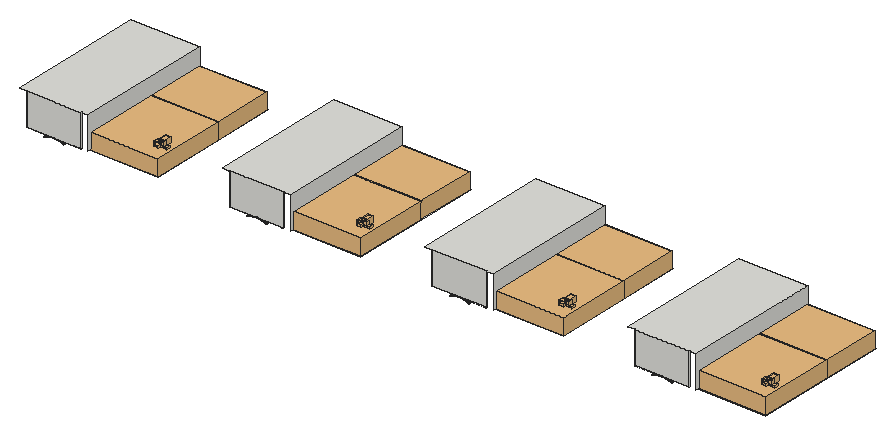
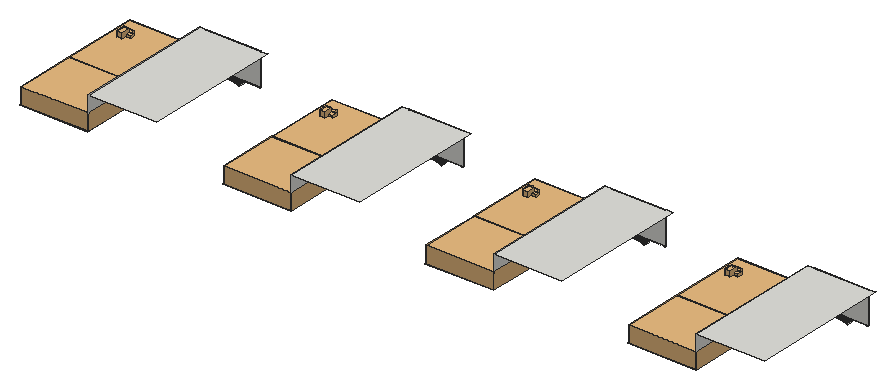
# SketchUp Ruby script. Lengths in inches.
U = 1.inch
M = Sketchup.active_model
def pt(a) = Geom::Point3d.new(a.map { |v| v * U })
def face(e, loops, mat)
  f = e.add_face(loops[0].map { |a| pt(a) })
  loops[1..].each { |l| e.add_face(l.map { |a| pt(a) }).erase! }
  f.material = f.back_material = mat if mat
  f
end
# faces: each face lists its corners as indices into pts; further lists are holes
def faces(e, pts, list, mat = nil) = list.each { |f| face(e, (f[0].is_a?(Array) ? f : [f]).map { |l| l.map { |i| pts[i] } }, mat) }
# xy, xz, yz: faces in a plane at the given z, y or x. An outline is a flat list of corners, or four numbers for a rectangle; further outlines are holes
def ring(l) = l.size == 4 ? [[l[0], l[1]], [l[2], l[1]], [l[2], l[3]], [l[0], l[3]]] : l.each_slice(2).to_a
def flat(e, list, mat, &to3) = list.each { |f| face(e, (f[0].is_a?(Array) ? f : [f]).map { |l| ring(l).map { |u, v| to3.(u, v) } }, mat) }
def xy(e, z, list, mat = nil) = flat(e, list, mat) { |x, y| [x, y, z] }
def xz(e, y, list, mat = nil) = flat(e, list, mat) { |x, z| [x, y, z] }
def yz(e, x, list, mat = nil) = flat(e, list, mat) { |y, z| [x, y, z] }
def lines(e, pts, list) = list.each { |a, b| e.add_line(pt(pts[a]), pt(pts[b])) }
# prism: a flat outline (further loops are holes) pulled along v
def prism(e, loops, v, mat = nil)
  f = face(e, loops, mat); d = Geom::Vector3d.new(v.map { |x| x * U })
  f.pushpull(f.normal.samedirection?(d) ? d.length : -d.length)
end
def box(e, o, s, mat = nil) = prism(e, [[o, [o[0] + s[0], o[1], o[2]], [o[0] + s[0], o[1] + s[1], o[2]], [o[0], o[1] + s[1], o[2]]]], [0, 0, s[2]], mat)
def at(x, y, z, deg = 0) = Geom::Transformation.translation(pt([x, y, z])) * Geom::Transformation.rotation(ORIGIN, Z_AXIS, deg.degrees)
def axes(o, x, y, z) = Geom::Transformation.new([*x, 0, *y, 0, *z, 0, *pt(o).to_a, 1])
def part(name) = M.definitions.add(name)
# library, detail: a bought-in or finely detailed component or shape, given as its bounding box
def library(name, o, s) = part(name).tap { |d| box(d.entities, o, s) }
def detail(e, o, s) = box(e.add_group.entities, o, s)
def put(e, d, t, mat = nil) = e.add_instance(d, t).tap { |i| i.material = mat if mat }
def group(e, t, mat = nil) = e.add_group.tap { |g| g.transformation = t; g.material = mat if mat }.entities
root = M.entities
M.materials.add("POT_TEXTURE_1").color = [172, 172, 172]
M.materials.add("soil1").color = [68, 55, 47]
c1 = library("Group\#96",[-662.41,217.3,320.04],[397.32,658.3,1732.06])
c2 = library("Group\#98",[-299.2,181.55,262.58],[360.65,735.71,1258.34])
c3 = library("Group\#93",[-1038.76,656.55,345.34],[733.18,460.51,2065.7])
c4 = library("Group\#91",[-445.29,890.31,329.28],[284.3,304.08,2023.29])
c5 = library("Group\#94",[-733.48,439.625,202.64],[456.28,533.12,1536.78])
c6 = library("Group\#97",[-455.56,899.32,410.78],[341.21,610.33,1581.5])
c7 = library("Group\#90",[-516.34,626.77,-4.5625],[517.73,515.95,418.98])
c8 = library("Group\#95",[-249.24,914.85,310.18],[345.55,647.95,1307.93])
c9 = library("Group\#92",[-277.97,488.68,287.26],[362.84,405.94,1768.54])
c10 = library("Group\#89",[-468.76,669.89,380.1875],[424.36,427.47,41.99])
c11 = part("Potted broadleaf plant")
put(c11.entities,c1,at(1038.76,-181.55,4.5625))
put(c11.entities,c2,at(1038.76,-181.55,4.5625))
put(c11.entities,c3,at(1038.76,-181.55,4.5625))
put(c11.entities,c4,at(1038.76,-181.55,4.5625))
put(c11.entities,c5,at(1038.76,-181.55,4.5625))
put(c11.entities,c6,at(1038.76,-181.55,4.5625))
put(c11.entities,c7,at(1038.76,-181.55,4.5625),"POT_TEXTURE_1")
put(c11.entities,c8,at(1038.76,-181.55,4.5625))
put(c11.entities,c9,at(1038.76,-181.55,4.5625))
put(c11.entities,c10,at(1038.76,-181.55,4.5625),"soil1")
c12 = library("Glass Railing\#2",[-0.5,-0.75,0],[149.1875,165.51,35.5])
c13 = library("Glass Railing\#3",[-148.4375,-0.5,0],[149.1875,132.1875,35.5])
xy(root,270.89,[[159.1,224.6875,215.92,225.16],[222.08,224.6875,278.75,225.16],[603.1,224.6875,659.92,225.16],[666.08,224.6875,722.75,225.16],[1047.1,224.6875,1103.92,225.16],
  [1110.08,224.6875,1166.75,225.16],[1491.1,224.6875,1547.92,225.16],[1554.08,224.6875,1610.75,225.16]])
xy(root,271,[[218.38,224.6875,219,225.16],[219,224.6875,219.61,225.16],[662.38,224.6875,663,225.16],[663,224.6875,663.61,225.16],[1106.38,224.6875,1107,225.16],
  [1107,224.6875,1107.61,225.16],[1550.38,224.6875,1551,225.16],[1551,224.6875,1551.61,225.16],[218.38,225.16,219,236.25],[219,225.16,219.61,236.25],
  [662.38,225.16,663,236.25],[663,225.16,663.61,236.25],[1106.38,225.16,1107,236.25],[1107,225.16,1107.61,236.25],[1550.38,225.16,1551,236.25],
  [1551,225.16,1551.61,236.25],[294,229.25,444,529.25],[738,229.25,888,529.25],[1182,229.25,1332,529.25],[1626,229.25,1776,529.25]])
xy(root,271.37,[[159.1,224.6875,215.92,225.16],[215.92,224.6875,222.08,225.16],[222.08,224.6875,278.75,225.16],[603.1,224.6875,659.92,225.16],[659.92,224.6875,666.08,225.16],
  [666.08,224.6875,722.75,225.16],[1047.1,224.6875,1103.92,225.16],[1103.92,224.6875,1110.08,225.16],[1110.08,224.6875,1166.75,225.16],[1491.1,224.6875,1547.92,225.16],
  [1547.92,224.6875,1554.08,225.16],[1554.08,224.6875,1610.75,225.16]])
xy(root,342,[[144,224.6875,158.625,224.6875,158.625,225.16,159.1,225.16,159.1,224.6875,278.75,224.6875,278.75,225.16,279.22,225.16,279.22,224.6875,294,224.6875,294,529.25,144,529.25],[588,224.6875,602.625,224.6875,602.625,225.16,603.1,225.16,603.1,224.6875,722.75,224.6875,722.75,225.16,723.22,225.16,723.22,224.6875,738,224.6875,738,529.25,588,529.25],[1032,224.6875,1046.625,224.6875,1046.625,225.16,1047.1,225.16,1047.1,224.6875,1166.75,224.6875,1166.75,225.16,1167.22,225.16,1167.22,224.6875,1182,224.6875,1182,529.25,1032,529.25],[1476,224.6875,1490.625,224.6875,1490.625,225.16,1491.1,225.16,1491.1,224.6875,1610.75,224.6875,1610.75,225.16,1611.22,225.16,1611.22,224.6875,1626,224.6875,1626,529.25,1476,529.25]])
xz(root,224.6875,[[215.92,270.89,222.08,270.89,222.05,270.9,220.83,270.96,219.61,271,218.38,271,217.77,270.98,217.15,270.96,216.53,270.93],[659.92,270.89,666.08,270.89,666.05,270.9,664.83,270.96,663.61,271,662.38,271,661.77,270.98,661.15,270.96,660.53,270.93],[1103.92,270.89,1110.08,270.89,1110.05,270.9,1108.83,270.96,1107.61,271,1106.38,271,1105.77,270.98,1105.15,270.96,1104.53,270.93],[1547.92,270.89,1554.08,270.89,1554.05,270.9,1552.83,270.96,1551.61,271,1550.38,271,1549.77,270.98,1549.15,270.96,1548.53,270.93],[159.1,271.37,278.75,342],
  [603.1,271.37,722.75,342],[1047.1,271.37,1166.75,342],[1491.1,271.37,1610.75,342]])
yz(root,159.1,[[224.6875,271.37,225.16,342]])
yz(root,278.75,[[224.6875,271.37,225.16,342]])
yz(root,294,[[224.6875,271,529.25,342]])
yz(root,603.1,[[224.6875,271.37,225.16,342]])
yz(root,722.75,[[224.6875,271.37,225.16,342]])
yz(root,738,[[224.6875,271,529.25,342]])
yz(root,1047.1,[[224.6875,271.37,225.16,342]])
yz(root,1166.75,[[224.6875,271.37,225.16,342]])
yz(root,1182,[[224.6875,271,529.25,342]])
yz(root,1491.1,[[224.6875,271.37,225.16,342]])
yz(root,1610.75,[[224.6875,271.37,225.16,342]])
yz(root,1626,[[224.6875,271,529.25,342]])
p = [[241.22,236.25,265.14],[241.22,224.6875,265.14],[240.68,224.6875,265.43],[240.68,236.25,265.43],[685.22,236.25,265.14],[685.22,224.6875,265.14],
  [684.68,224.6875,265.43],[684.68,236.25,265.43],[1129.22,236.25,265.14],[1129.22,224.6875,265.14],[1128.68,224.6875,265.43],[1128.68,236.25,265.43],
  [1573.22,236.25,265.14],[1573.22,224.6875,265.14],[1572.68,224.6875,265.43],[1572.68,236.25,265.43],[197.69,236.25,265.62],[197.69,224.6875,265.62],
  [197.15,224.6875,265.32],[197.15,236.25,265.32],[641.69,236.25,265.62],[641.69,224.6875,265.62],[641.15,224.6875,265.32],[641.15,236.25,265.32],
  [1085.69,236.25,265.62],[1085.69,224.6875,265.62],[1085.15,224.6875,265.32],[1085.15,236.25,265.32],[1529.69,236.25,265.62],[1529.69,224.6875,265.62],
  [1529.15,224.6875,265.32],[1529.15,236.25,265.32],[240.15,224.6875,265.72],[240.15,236.25,265.72],[684.15,224.6875,265.72],[684.15,236.25,265.72],
  [1128.15,224.6875,265.72],[1128.15,236.25,265.72],[1572.15,224.6875,265.72],[1572.15,236.25,265.72],[198.24,236.25,265.91],[198.24,224.6875,265.91],
  [642.24,236.25,265.91],[642.24,224.6875,265.91],[1086.24,236.25,265.91],[1086.24,224.6875,265.91],[1530.24,236.25,265.91],[1530.24,224.6875,265.91],
  [239.6,224.6875,266.01],[239.6,236.25,266.01],[683.6,224.6875,266.01],[683.6,236.25,266.01],[1127.6,224.6875,266.01],[1127.6,236.25,266.01],
  [1571.6,224.6875,266.01],[1571.6,236.25,266.01],[198.79,236.25,266.1875],[198.79,224.6875,266.1875],[642.79,236.25,266.1875],[642.79,224.6875,266.1875],
  [1086.79,236.25,266.1875],[1086.79,224.6875,266.1875],[1530.79,236.25,266.1875],[1530.79,224.6875,266.1875],[239.06,224.6875,266.28],[239.06,236.25,266.28],
  [683.06,224.6875,266.28],[683.06,236.25,266.28],[1127.06,224.6875,266.28],[1127.06,236.25,266.28],[1571.06,224.6875,266.28],[1571.06,236.25,266.28],
  [199.34,236.25,266.46],[199.34,224.6875,266.46],[643.34,236.25,266.46],[643.34,224.6875,266.46],[1087.34,236.25,266.46],[1087.34,224.6875,266.46],
  [1531.34,236.25,266.46],[1531.34,224.6875,266.46],[238.51,224.6875,266.55],[238.51,236.25,266.55],[682.51,224.6875,266.55],[682.51,236.25,266.55],
  [1126.51,224.6875,266.55],[1126.51,236.25,266.55],[1570.51,224.6875,266.55],[1570.51,236.25,266.55],[199.89,236.25,266.73],[199.89,224.6875,266.73],
  [643.89,236.25,266.73],[643.89,224.6875,266.73],[1087.89,236.25,266.73],[1087.89,224.6875,266.73],[1531.89,236.25,266.73],[1531.89,224.6875,266.73],
  [237.96,224.6875,266.8125],[237.96,236.25,266.8125],[681.96,224.6875,266.8125],[681.96,236.25,266.8125],[1125.96,224.6875,266.8125],[1125.96,236.25,266.8125],
  [1569.96,224.6875,266.8125],[1569.96,236.25,266.8125],[200.45,236.25,266.99],[200.45,224.6875,266.99],[644.45,236.25,266.99],[644.45,224.6875,266.99],
  [1088.45,236.25,266.99],[1088.45,224.6875,266.99],[1532.45,236.25,266.99],[1532.45,224.6875,266.99],[237.4,224.6875,267.07],[237.4,236.25,267.07],
  [681.4,224.6875,267.07],[681.4,236.25,267.07],[1125.4,224.6875,267.07],[1125.4,236.25,267.07],[1569.4,224.6875,267.07],[1569.4,236.25,267.07],
  [201.02,236.25,267.24],[201.02,224.6875,267.24],[645.02,236.25,267.24],[645.02,224.6875,267.24],[1089.02,236.25,267.24],[1089.02,224.6875,267.24],
  [1533.02,236.25,267.24],[1533.02,224.6875,267.24],[236.84,224.6875,267.3125],[236.84,236.25,267.3125],[680.84,224.6875,267.3125],[680.84,236.25,267.3125],
  [1124.84,224.6875,267.3125],[1124.84,236.25,267.3125],[1568.84,224.6875,267.3125],[1568.84,236.25,267.3125],[201.58,236.25,267.48],[201.58,224.6875,267.48],
  [645.58,236.25,267.48],[645.58,224.6875,267.48],[1089.58,236.25,267.48],[1089.58,224.6875,267.48],[1533.58,236.25,267.48],[1533.58,224.6875,267.48],
  [236.28,224.6875,267.55],[236.28,236.25,267.55],[680.28,224.6875,267.55],[680.28,236.25,267.55],[1124.28,224.6875,267.55],[1124.28,236.25,267.55],
  [1568.28,224.6875,267.55],[1568.28,236.25,267.55],[202.15,236.25,267.72],[202.15,224.6875,267.72],[646.15,236.25,267.72],[646.15,224.6875,267.72],
  [1090.15,236.25,267.72],[1090.15,224.6875,267.72],[1534.15,236.25,267.72],[1534.15,224.6875,267.72],[235.71,224.6875,267.78],[235.71,236.25,267.78],
  [679.71,224.6875,267.78],[679.71,236.25,267.78],[1123.71,224.6875,267.78],[1123.71,236.25,267.78],[1567.71,224.6875,267.78],[1567.71,236.25,267.78],
  [202.73,236.25,267.94],[202.73,224.6875,267.94],[646.73,236.25,267.94],[646.73,224.6875,267.94],[1090.73,236.25,267.94],[1090.73,224.6875,267.94],
  [1534.73,236.25,267.94],[1534.73,224.6875,267.94],[235.14,224.6875,268.01],[235.14,236.25,268.01],[679.14,224.6875,268.01],[679.14,236.25,268.01],
  [1123.14,224.6875,268.01],[1123.14,236.25,268.01],[1567.14,224.6875,268.01],[1567.14,236.25,268.01],[203.3,236.25,268.16],[203.3,224.6875,268.16],
  [647.3,236.25,268.16],[647.3,224.6875,268.16],[1091.3,236.25,268.16],[1091.3,224.6875,268.16],[1535.3,236.25,268.16],[1535.3,224.6875,268.16],
  [234.57,224.6875,268.22],[234.57,236.25,268.22],[678.57,224.6875,268.22],[678.57,236.25,268.22],[1122.57,224.6875,268.22],[1122.57,236.25,268.22],
  [1566.57,224.6875,268.22],[1566.57,236.25,268.22],[203.88,236.25,268.375],[203.88,224.6875,268.375],[233.99,224.6875,268.43],[233.99,236.25,268.43],
  [647.88,236.25,268.375],[647.88,224.6875,268.375],[677.99,224.6875,268.43],[677.99,236.25,268.43],[1091.88,236.25,268.375],[1091.88,224.6875,268.375],
  [1121.99,224.6875,268.43],[1121.99,236.25,268.43],[1535.88,236.25,268.375],[1535.88,224.6875,268.375],[1565.99,224.6875,268.43],[1565.99,236.25,268.43],
  [204.46,236.25,268.58],[204.46,224.6875,268.58],[233.42,224.6875,268.63],[233.42,236.25,268.63],[648.46,236.25,268.58],[648.46,224.6875,268.58],
  [677.42,224.6875,268.63],[677.42,236.25,268.63],[1092.46,236.25,268.58],[1092.46,224.6875,268.58],[1121.42,224.6875,268.63],[1121.42,236.25,268.63],
  [1536.46,236.25,268.58],[1536.46,224.6875,268.58],[1565.42,224.6875,268.63],[1565.42,236.25,268.63],[205.05,236.25,268.78],[205.05,224.6875,268.78],
  [232.84,224.6875,268.82],[232.84,236.25,268.82],[649.05,236.25,268.78],[649.05,224.6875,268.78],[676.84,224.6875,268.82],[676.84,236.25,268.82],
  [1093.05,236.25,268.78],[1093.05,224.6875,268.78],[1120.84,224.6875,268.82],[1120.84,236.25,268.82],[1537.05,236.25,268.78],[1537.05,224.6875,268.78],
  [1564.84,224.6875,268.82],[1564.84,236.25,268.82],[205.64,236.25,268.96],[205.64,224.6875,268.96],[232.25,224.6875,269],[232.25,236.25,269],
  [649.64,236.25,268.96],[649.64,224.6875,268.96],[676.25,224.6875,269],[676.25,236.25,269],[1093.64,236.25,268.96],[1093.64,224.6875,268.96],
  [1120.25,224.6875,269],[1120.25,236.25,269],[1537.64,236.25,268.96],[1537.64,224.6875,268.96],[1564.25,224.6875,269],[1564.25,236.25,269],
  [206.23,236.25,269.14],[206.23,224.6875,269.14],[231.67,224.6875,269.18],[231.67,236.25,269.18],[650.23,236.25,269.14],[650.23,224.6875,269.14],
  [675.67,224.6875,269.18],[675.67,236.25,269.18],[1094.23,236.25,269.14],[1094.23,224.6875,269.14],[1119.67,224.6875,269.18],[1119.67,236.25,269.18],
  [1538.23,236.25,269.14],[1538.23,224.6875,269.14],[1563.67,224.6875,269.18],[1563.67,236.25,269.18],[206.82,236.25,269.31],[206.82,224.6875,269.31],
  [650.82,236.25,269.31],[650.82,224.6875,269.31],[1094.82,236.25,269.31],[1094.82,224.6875,269.31],[1538.82,236.25,269.31],[1538.82,224.6875,269.31],
  [231.08,224.6875,269.35],[231.08,236.25,269.35],[675.08,224.6875,269.35],[675.08,236.25,269.35],[1119.08,224.6875,269.35],[1119.08,236.25,269.35],
  [1563.08,224.6875,269.35],[1563.08,236.25,269.35],[207.41,236.25,269.48],[207.41,224.6875,269.48],[230.49,224.6875,269.51],[230.49,236.25,269.51],
  [651.41,236.25,269.48],[651.41,224.6875,269.48],[674.49,224.6875,269.51],[674.49,236.25,269.51],[1095.41,236.25,269.48],[1095.41,224.6875,269.48],
  [1118.49,224.6875,269.51],[1118.49,236.25,269.51],[1539.41,236.25,269.48],[1539.41,224.6875,269.48],[1562.49,224.6875,269.51],[1562.49,236.25,269.51],
  [208.01,236.25,269.63],[208.01,224.6875,269.63],[229.9,224.6875,269.66],[229.9,236.25,269.66],[652.01,236.25,269.63],[652.01,224.6875,269.63],
  [673.9,224.6875,269.66],[673.9,236.25,269.66],[1096.01,236.25,269.63],[1096.01,224.6875,269.63],[1117.9,224.6875,269.66],[1117.9,236.25,269.66],
  [1540.01,236.25,269.63],[1540.01,224.6875,269.63],[1561.9,224.6875,269.66],[1561.9,236.25,269.66],[208.61,236.25,269.78],[208.61,224.6875,269.78],
  [652.61,236.25,269.78],[652.61,224.6875,269.78],[1096.61,236.25,269.78],[1096.61,224.6875,269.78],[1540.61,236.25,269.78],[1540.61,224.6875,269.78],
  [229.3,224.6875,269.81],[229.3,236.25,269.81],[673.3,224.6875,269.81],[673.3,236.25,269.81],[1117.3,224.6875,269.81],[1117.3,236.25,269.81],
  [1561.3,224.6875,269.81],[1561.3,236.25,269.81],[209.21,236.25,269.92],[209.21,224.6875,269.92],[228.71,224.6875,269.94],[228.71,236.25,269.94],
  [653.21,236.25,269.92],[653.21,224.6875,269.92],[672.71,224.6875,269.94],[672.71,236.25,269.94],[1097.21,236.25,269.92],[1097.21,224.6875,269.92],
  [1116.71,224.6875,269.94],[1116.71,236.25,269.94],[1541.21,236.25,269.92],[1541.21,224.6875,269.92],[1560.71,224.6875,269.94],[1560.71,236.25,269.94],
  [209.8125,236.25,270.05],[209.8125,224.6875,270.05],[228.11,224.6875,270.07],[228.11,236.25,270.07],[653.8125,236.25,270.05],[653.8125,224.6875,270.05],
  [672.11,224.6875,270.07],[672.11,236.25,270.07],[1097.8125,236.25,270.05],[1097.8125,224.6875,270.05],[1116.11,224.6875,270.07],[1116.11,236.25,270.07],
  [1541.8125,236.25,270.05],[1541.8125,224.6875,270.05],[1560.11,224.6875,270.07],[1560.11,236.25,270.07],[210.42,236.25,270.17],[210.42,224.6875,270.17],
  [654.42,236.25,270.17],[654.42,224.6875,270.17],[1098.42,236.25,270.17],[1098.42,224.6875,270.17],[1542.42,236.25,270.17],[1542.42,224.6875,270.17],
  [227.51,224.6875,270.1875],[227.51,236.25,270.1875],[671.51,224.6875,270.1875],[671.51,236.25,270.1875],[1115.51,224.6875,270.1875],[1115.51,236.25,270.1875],
  [1559.51,224.6875,270.1875],[1559.51,236.25,270.1875],[211.02,236.25,270.29],[211.02,224.6875,270.29],[226.91,224.6875,270.3],[226.91,236.25,270.3],
  [655.02,236.25,270.29],[655.02,224.6875,270.29],[670.91,224.6875,270.3],[670.91,236.25,270.3],[1099.02,236.25,270.29],[1099.02,224.6875,270.29],
  [1114.91,224.6875,270.3],[1114.91,236.25,270.3],[1543.02,236.25,270.29],[1543.02,224.6875,270.29],[1558.91,224.6875,270.3],[1558.91,236.25,270.3],
  [211.63,236.25,270.39],[211.63,224.6875,270.39],[226.3,224.6875,270.4],[226.3,236.25,270.4],[655.63,236.25,270.39],[655.63,224.6875,270.39],
  [670.3,224.6875,270.4],[670.3,236.25,270.4],[1099.63,236.25,270.39],[1099.63,224.6875,270.39],[1114.3,224.6875,270.4],[1114.3,236.25,270.4],
  [1543.63,236.25,270.39],[1543.63,224.6875,270.39],[1558.3,224.6875,270.4],[1558.3,236.25,270.4],[212.24,236.25,270.49],[212.24,224.6875,270.49],
  [225.7,224.6875,270.5],[225.7,236.25,270.5],[656.24,236.25,270.49],[656.24,224.6875,270.49],[669.7,224.6875,270.5],[669.7,236.25,270.5],
  [1100.24,236.25,270.49],[1100.24,224.6875,270.49],[1113.7,224.6875,270.5],[1113.7,236.25,270.5],[1544.24,236.25,270.49],[1544.24,224.6875,270.49],
  [1557.7,224.6875,270.5],[1557.7,236.25,270.5],[212.85,236.25,270.58],[212.85,224.6875,270.58],[225.1,224.6875,270.59],[225.1,236.25,270.59],
  [656.85,236.25,270.58],[656.85,224.6875,270.58],[669.1,224.6875,270.59],[669.1,236.25,270.59],[1100.85,236.25,270.58],[1100.85,224.6875,270.58],
  [1113.1,224.6875,270.59],[1113.1,236.25,270.59],[1544.85,236.25,270.58],[1544.85,224.6875,270.58],[1557.1,224.6875,270.59],[1557.1,236.25,270.59],
  [213.46,236.25,270.66],[213.46,224.6875,270.66],[224.49,224.6875,270.66],[224.49,236.25,270.66],[657.46,236.25,270.66],[657.46,224.6875,270.66],
  [668.49,224.6875,270.66],[668.49,236.25,270.66],[1101.46,236.25,270.66],[1101.46,224.6875,270.66],[1112.49,224.6875,270.66],[1112.49,236.25,270.66],
  [1545.46,236.25,270.66],[1545.46,224.6875,270.66],[1556.49,224.6875,270.66],[1556.49,236.25,270.66],[214.08,236.25,270.73],[214.08,224.6875,270.73],
  [214.6875,236.25,270.79],[214.6875,224.6875,270.79],[223.88,236.25,270.73],[223.88,224.6875,270.73],[223.27,224.6875,270.8],[223.27,236.25,270.8],
  [658.08,236.25,270.73],[658.08,224.6875,270.73],[658.6875,236.25,270.79],[658.6875,224.6875,270.79],[667.88,236.25,270.73],[667.88,224.6875,270.73],
  [667.27,224.6875,270.8],[667.27,236.25,270.8],[1102.08,236.25,270.73],[1102.08,224.6875,270.73],[1102.6875,236.25,270.79],[1102.6875,224.6875,270.79],
  [1111.88,236.25,270.73],[1111.88,224.6875,270.73],[1111.27,224.6875,270.8],[1111.27,236.25,270.8],[1546.08,236.25,270.73],[1546.08,224.6875,270.73],
  [1546.6875,236.25,270.79],[1546.6875,224.6875,270.79],[1555.88,236.25,270.73],[1555.88,224.6875,270.73],[1555.27,224.6875,270.8],[1555.27,236.25,270.8],
  [215.3,236.25,270.85],[215.3,224.6875,270.85],[215.92,225.16,270.89],[215.92,224.6875,270.89],[215.92,236.25,270.89],[222.66,224.6875,270.85],
  [222.66,236.25,270.85],[659.3,236.25,270.85],[659.3,224.6875,270.85],[659.92,225.16,270.89],[659.92,224.6875,270.89],[659.92,236.25,270.89],
  [666.66,224.6875,270.85],[666.66,236.25,270.85],[1103.3,236.25,270.85],[1103.3,224.6875,270.85],[1103.92,225.16,270.89],[1103.92,224.6875,270.89],
  [1103.92,236.25,270.89],[1110.66,224.6875,270.85],[1110.66,236.25,270.85],[1547.3,236.25,270.85],[1547.3,224.6875,270.85],[1547.92,225.16,270.89],
  [1547.92,224.6875,270.89],[1547.92,236.25,270.89],[1554.66,224.6875,270.85],[1554.66,236.25,270.85],[216.53,224.6875,270.93],[216.53,225.16,270.93],
  [217.15,224.6875,270.96],[217.15,225.16,270.96],[221.44,224.6875,270.93],[220.83,224.6875,270.96],[220.83,225.16,270.96],[221.44,225.16,270.93],
  [222.05,224.6875,270.9],[222.05,225.16,270.9],[222.08,224.6875,270.89],[222.08,225.16,270.89],[222.05,236.25,270.9],[660.53,224.6875,270.93],
  [660.53,225.16,270.93],[661.15,224.6875,270.96],[661.15,225.16,270.96],[665.44,224.6875,270.93],[664.83,224.6875,270.96],[664.83,225.16,270.96],
  [665.44,225.16,270.93],[666.05,224.6875,270.9],[666.05,225.16,270.9],[666.08,224.6875,270.89],[666.08,225.16,270.89],[666.05,236.25,270.9],
  [1104.53,224.6875,270.93],[1104.53,225.16,270.93],[1105.15,224.6875,270.96],[1105.15,225.16,270.96],[1109.44,224.6875,270.93],[1108.83,224.6875,270.96],
  [1108.83,225.16,270.96],[1109.44,225.16,270.93],[1110.05,224.6875,270.9],[1110.05,225.16,270.9],[1110.08,224.6875,270.89],[1110.08,225.16,270.89],
  [1110.05,236.25,270.9],[1548.53,224.6875,270.93],[1548.53,225.16,270.93],[1549.15,224.6875,270.96],[1549.15,225.16,270.96],[1553.44,224.6875,270.93],
  [1552.83,224.6875,270.96],[1552.83,225.16,270.96],[1553.44,225.16,270.93],[1554.05,224.6875,270.9],[1554.05,225.16,270.9],[1554.08,224.6875,270.89],
  [1554.08,225.16,270.89],[1554.05,236.25,270.9],[216.53,236.25,270.93],[217.15,236.25,270.96],[221.44,236.25,270.93],[220.83,236.25,270.96],
  [660.53,236.25,270.93],[661.15,236.25,270.96],[665.44,236.25,270.93],[664.83,236.25,270.96],[1104.53,236.25,270.93],[1105.15,236.25,270.96],
  [1109.44,236.25,270.93],[1108.83,236.25,270.96],[1548.53,236.25,270.93],[1549.15,236.25,270.96],[1553.44,236.25,270.93],[1552.83,236.25,270.96],
  [217.77,224.6875,270.98],[217.77,225.16,270.98],[218.38,224.6875,271],[218.38,225.16,271],[220.22,224.6875,270.98],[219.61,224.6875,271],
  [219.61,225.16,271],[220.22,225.16,270.98],[661.77,224.6875,270.98],[661.77,225.16,270.98],[662.38,224.6875,271],[662.38,225.16,271],
  [664.22,224.6875,270.98],[663.61,224.6875,271],[663.61,225.16,271],[664.22,225.16,270.98],[1105.77,224.6875,270.98],[1105.77,225.16,270.98],
  [1106.38,224.6875,271],[1106.38,225.16,271],[1108.22,224.6875,270.98],[1107.61,224.6875,271],[1107.61,225.16,271],[1108.22,225.16,270.98],
  [1549.77,224.6875,270.98],[1549.77,225.16,270.98],[1550.38,224.6875,271],[1550.38,225.16,271],[1552.22,224.6875,270.98],[1551.61,224.6875,271],
  [1551.61,225.16,271],[1552.22,225.16,270.98],[217.77,236.25,270.98],[218.38,236.25,271],[220.22,236.25,270.98],[219.61,236.25,271],
  [661.77,236.25,270.98],[662.38,236.25,271],[664.22,236.25,270.98],[663.61,236.25,271],[1105.77,236.25,270.98],[1106.38,236.25,271],
  [1108.22,236.25,270.98],[1107.61,236.25,271],[1549.77,236.25,270.98],[1550.38,236.25,271],[1552.22,236.25,270.98],[1551.61,236.25,271]]
faces(root,p,[[0,1,2,3],[4,5,6,7],[8,9,10,11],[12,13,14,15],[16,17,18,19],[20,21,22,23],[24,25,26,27],[28,29,30,31],
  [3,2,32,33],[7,6,34,35],[11,10,36,37],[15,14,38,39],[40,41,17,16],[42,43,21,20],[44,45,25,24],[46,47,29,28],
  [33,32,48,49],[35,34,50,51],[37,36,52,53],[39,38,54,55],[56,57,41,40],[58,59,43,42],[60,61,45,44],[62,63,47,46],
  [49,48,64,65],[51,50,66,67],[53,52,68,69],[55,54,70,71],[72,73,57,56],[74,75,59,58],[76,77,61,60],[78,79,63,62],
  [65,64,80,81],[67,66,82,83],[69,68,84,85],[71,70,86,87],[88,89,73,72],[90,91,75,74],[92,93,77,76],[94,95,79,78],
  [81,80,96,97],[83,82,98,99],[85,84,100,101],[87,86,102,103],[104,105,89,88],[106,107,91,90],[108,109,93,92],[110,111,95,94],
  [97,96,112,113],[99,98,114,115],[101,100,116,117],[103,102,118,119],[120,121,105,104],[122,123,107,106],[124,125,109,108],[126,127,111,110],
  [113,112,128,129],[115,114,130,131],[117,116,132,133],[119,118,134,135],[136,137,121,120],[138,139,123,122],[140,141,125,124],[142,143,127,126],
  [129,128,144,145],[131,130,146,147],[133,132,148,149],[135,134,150,151],[152,153,137,136],[154,155,139,138],[156,157,141,140],[158,159,143,142],
  [145,144,160,161],[147,146,162,163],[149,148,164,165],[151,150,166,167],[168,169,153,152],[170,171,155,154],[172,173,157,156],[174,175,159,158],
  [161,160,176,177],[163,162,178,179],[165,164,180,181],[167,166,182,183],[184,185,169,168],[186,187,171,170],[188,189,173,172],[190,191,175,174],
  [177,176,192,193],[179,178,194,195],[181,180,196,197],[183,182,198,199],[200,201,185,184],[193,192,202,203],[204,205,187,186],[195,194,206,207],
  [208,209,189,188],[197,196,210,211],[212,213,191,190],[199,198,214,215],[216,217,201,200],[203,202,218,219],[220,221,205,204],[207,206,222,223],
  [224,225,209,208],[211,210,226,227],[228,229,213,212],[215,214,230,231],[232,233,217,216],[219,218,234,235],[236,237,221,220],[223,222,238,239],
  [240,241,225,224],[227,226,242,243],[244,245,229,228],[231,230,246,247],[248,249,233,232],[235,234,250,251],[252,253,237,236],[239,238,254,255],
  [256,257,241,240],[243,242,258,259],[260,261,245,244],[247,246,262,263],[264,265,249,248],[251,250,266,267],[268,269,253,252],[255,254,270,271],
  [272,273,257,256],[259,258,274,275],[276,277,261,260],[263,262,278,279],[280,281,265,264],[282,283,269,268],[284,285,273,272],[286,287,277,276],
  [267,266,288,289],[271,270,290,291],[275,274,292,293],[279,278,294,295],[296,297,281,280],[289,288,298,299],[300,301,283,282],[291,290,302,303],
  [304,305,285,284],[293,292,306,307],[308,309,287,286],[295,294,310,311],[312,313,297,296],[299,298,314,315],[316,317,301,300],[303,302,318,319],
  [320,321,305,304],[307,306,322,323],[324,325,309,308],[311,310,326,327],[328,329,313,312],[330,331,317,316],[332,333,321,320],[334,335,325,324],
  [315,314,336,337],[319,318,338,339],[323,322,340,341],[327,326,342,343],[344,345,329,328],[337,336,346,347],[348,349,331,330],[339,338,350,351],
  [352,353,333,332],[341,340,354,355],[356,357,335,334],[343,342,358,359],[360,361,345,344],[347,346,362,363],[364,365,349,348],[351,350,366,367],
  [368,369,353,352],[355,354,370,371],[372,373,357,356],[359,358,374,375],[376,377,361,360],[378,379,365,364],[380,381,369,368],[382,383,373,372],
  [363,362,384,385],[367,366,386,387],[371,370,388,389],[375,374,390,391],[392,393,377,376],[385,384,394,395],[396,397,379,378],[387,386,398,399],
  [400,401,381,380],[389,388,402,403],[404,405,383,382],[391,390,406,407],[408,409,393,392],[395,394,410,411],[412,413,397,396],[399,398,414,415],
  [416,417,401,400],[403,402,418,419],[420,421,405,404],[407,406,422,423],[424,425,409,408],[411,410,426,427],[428,429,413,412],[415,414,430,431],
  [432,433,417,416],[419,418,434,435],[436,437,421,420],[423,422,438,439],[440,441,425,424],[427,426,442,443],[444,445,429,428],[431,430,446,447],
  [448,449,433,432],[435,434,450,451],[452,453,437,436],[439,438,454,455],[456,457,441,440],[443,442,458,459],[460,461,445,444],[447,446,462,463],
  [464,465,449,448],[451,450,466,467],[468,469,453,452],[455,454,470,471],[472,473,457,456],[474,475,473,472],[476,477,478,479],[459,458,477,476],
  [480,481,461,460],[482,483,481,480],[484,485,486,487],[463,462,485,484],[488,489,465,464],[490,491,489,488],[492,493,494,495],[467,466,493,492],
  [496,497,469,468],[498,499,497,496],[500,501,502,503],[471,470,501,500],[504,505,475,474],[506,507,505,504,508],[479,478,509,510],[511,512,483,482],
  [513,514,512,511,515],[487,486,516,517],[518,519,491,490],[520,521,519,518,522],[495,494,523,524],[525,526,499,498],[527,528,526,525,529],[503,502,530,531],
  [532,507,506,533],[534,532,533,535],[536,537,538,539],[540,536,539,541],[510,509,542,543,541,544],[542,540,541,543],[545,514,513,546],[547,545,546,548],
  [549,550,551,552],[553,549,552,554],[517,516,555,556,554,557],[555,553,554,556],[558,521,520,559],[560,558,559,561],[562,563,564,565],[566,562,565,567],
  [524,523,568,569,567,570],[568,566,567,569],[571,528,527,572],[573,571,572,574],[575,576,577,578],[579,575,578,580],[531,530,581,582,580,583],[581,579,580,582],
  [584,533,506,508],[585,535,533,584],[586,539,538,587],[544,541,539,586],[588,546,513,515],[589,548,546,588],[590,552,551,591],[557,554,552,590],
  [592,559,520,522],[593,561,559,592],[594,565,564,595],[570,567,565,594],[596,572,527,529],[597,574,572,596],[598,578,577,599],[583,580,578,598],
  [600,534,535,601],[602,600,601,603],[604,605,606,607],[537,604,607,538],[608,547,548,609],[610,608,609,611],[612,613,614,615],[550,612,615,551],
  [616,560,561,617],[618,616,617,619],[620,621,622,623],[563,620,623,564],[624,573,574,625],[626,624,625,627],[628,629,630,631],[576,628,631,577],
  [632,601,535,585],[633,603,601,632],[634,607,606,635],[587,538,607,634],[636,609,548,589],[637,611,609,636],[638,615,614,639],[591,551,615,638],
  [640,617,561,593],[641,619,617,640],[642,623,622,643],[595,564,623,642],[644,625,574,597],[645,627,625,644],[646,631,630,647],[599,577,631,646]])
put(root,c11,axes([401.3,287.84,271],[0,-0.0242,0],[0.0242,0,0],[0,0,0.01917]))
put(root,c11,axes([845.3,287.84,271],[0,-0.0242,0],[0.0242,0,0],[0,0,0.01917]))
put(root,c11,axes([1289.3,287.84,271],[0,-0.0242,0],[0.0242,0,0],[0,0,0.01917]))
put(root,c11,axes([1733.3,287.84,271],[0,-0.0242,0],[0.0242,0,0],[0,0,0.01917]))
put(root,c12,at(294,231.37,271))
put(root,c13,at(441.9375,396.125,271))
put(root,c12,at(738,231.37,271))
put(root,c13,at(885.9375,396.125,271))
put(root,c12,at(1182,231.37,271))
put(root,c13,at(1329.9375,396.125,271))
put(root,c12,at(1626,231.37,271))
put(root,c13,at(1773.9375,396.125,271))
